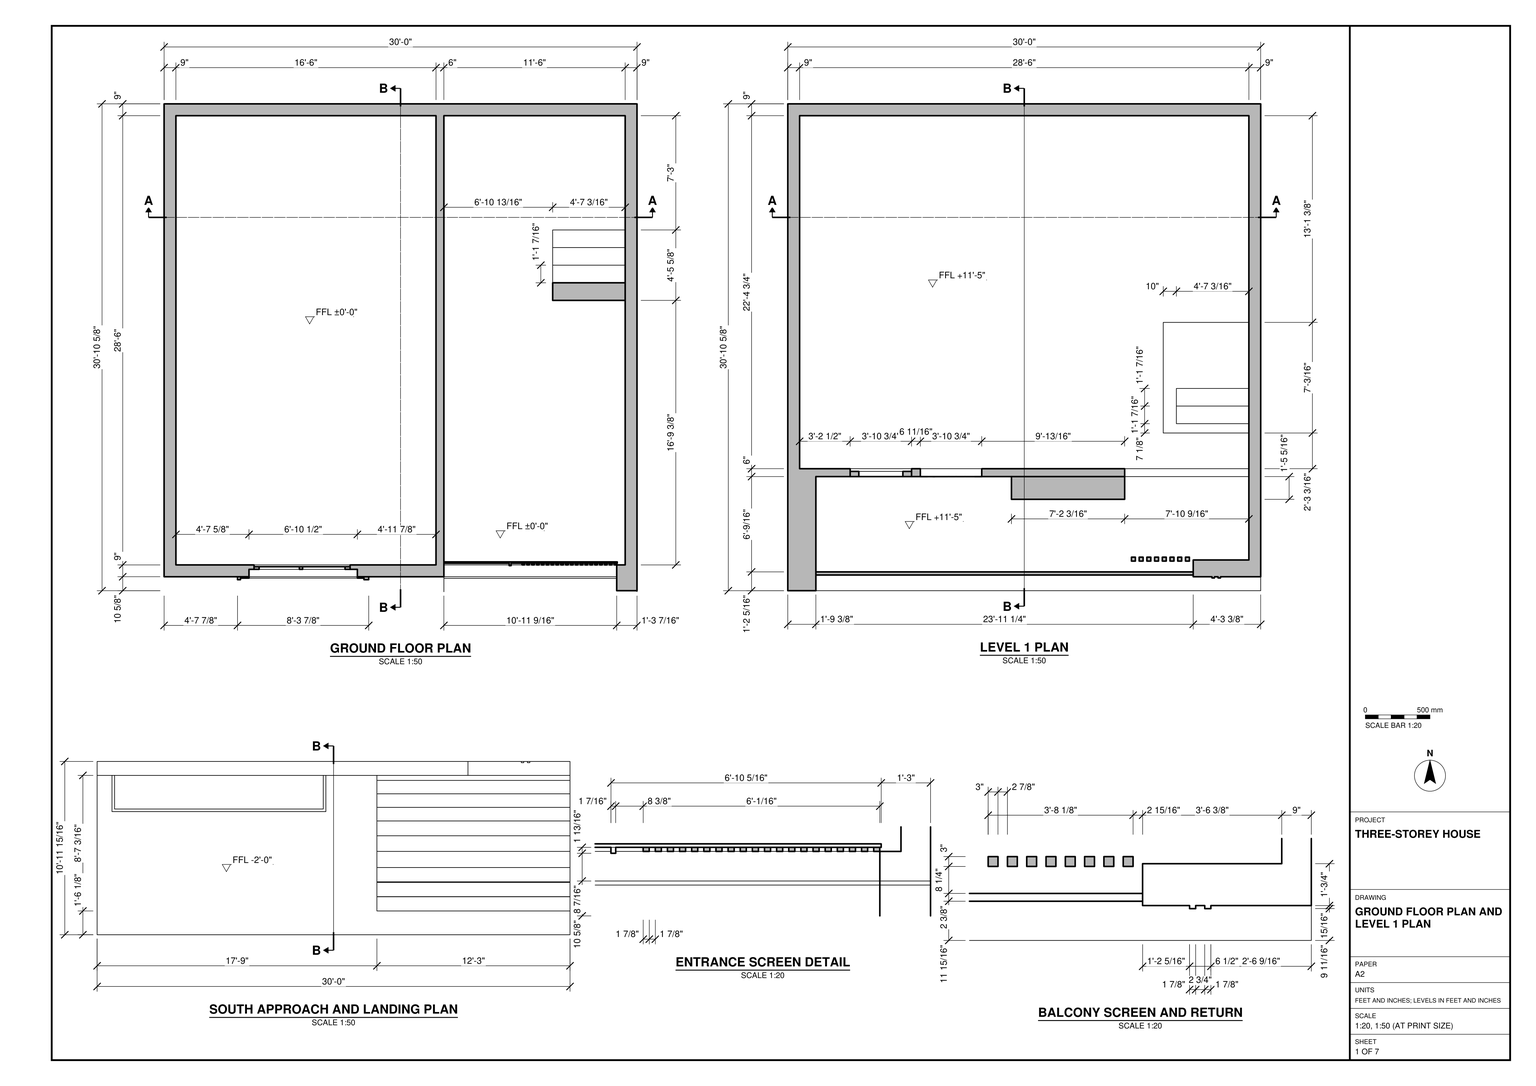
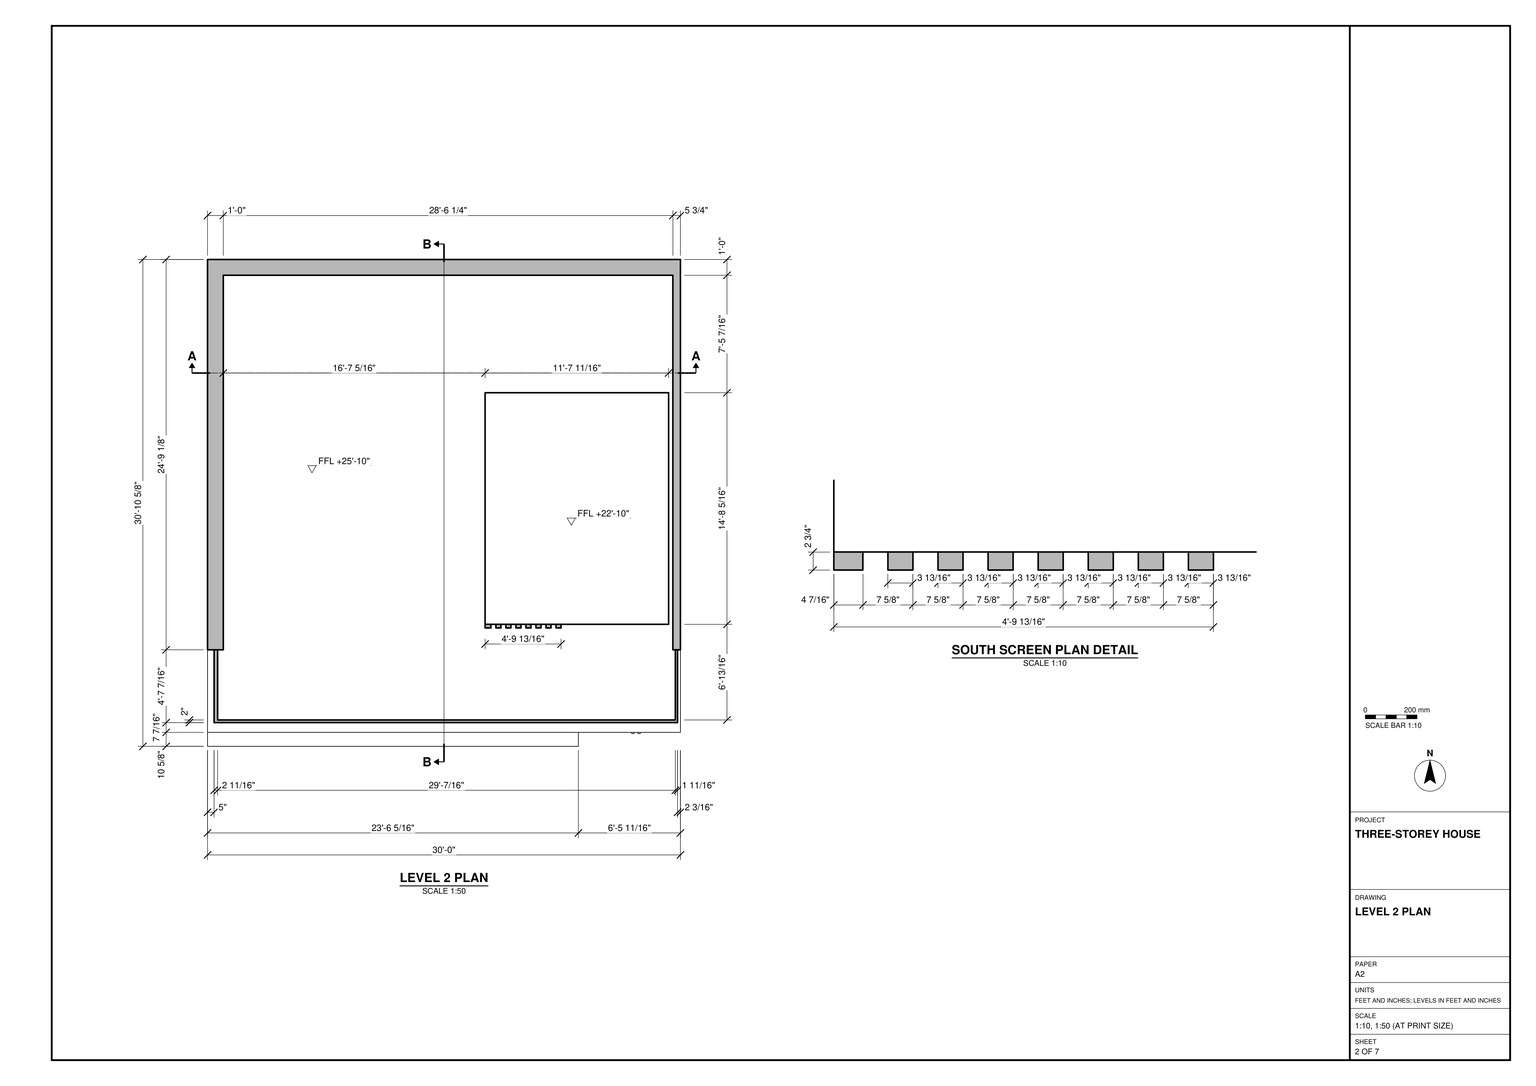
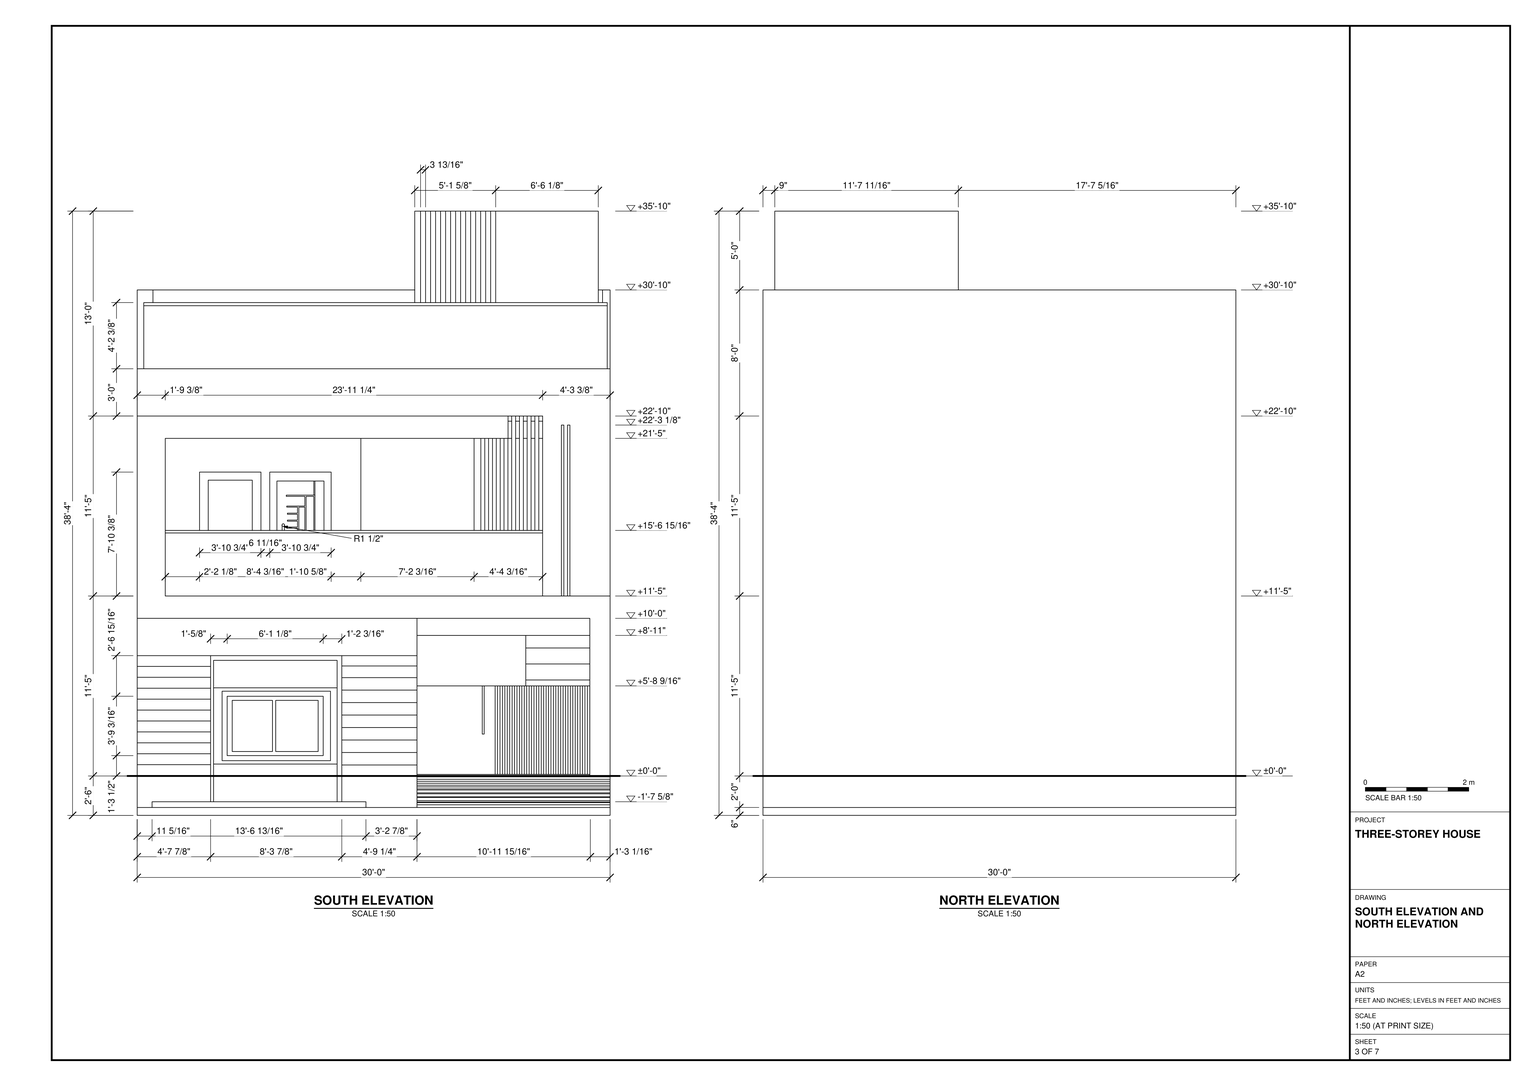
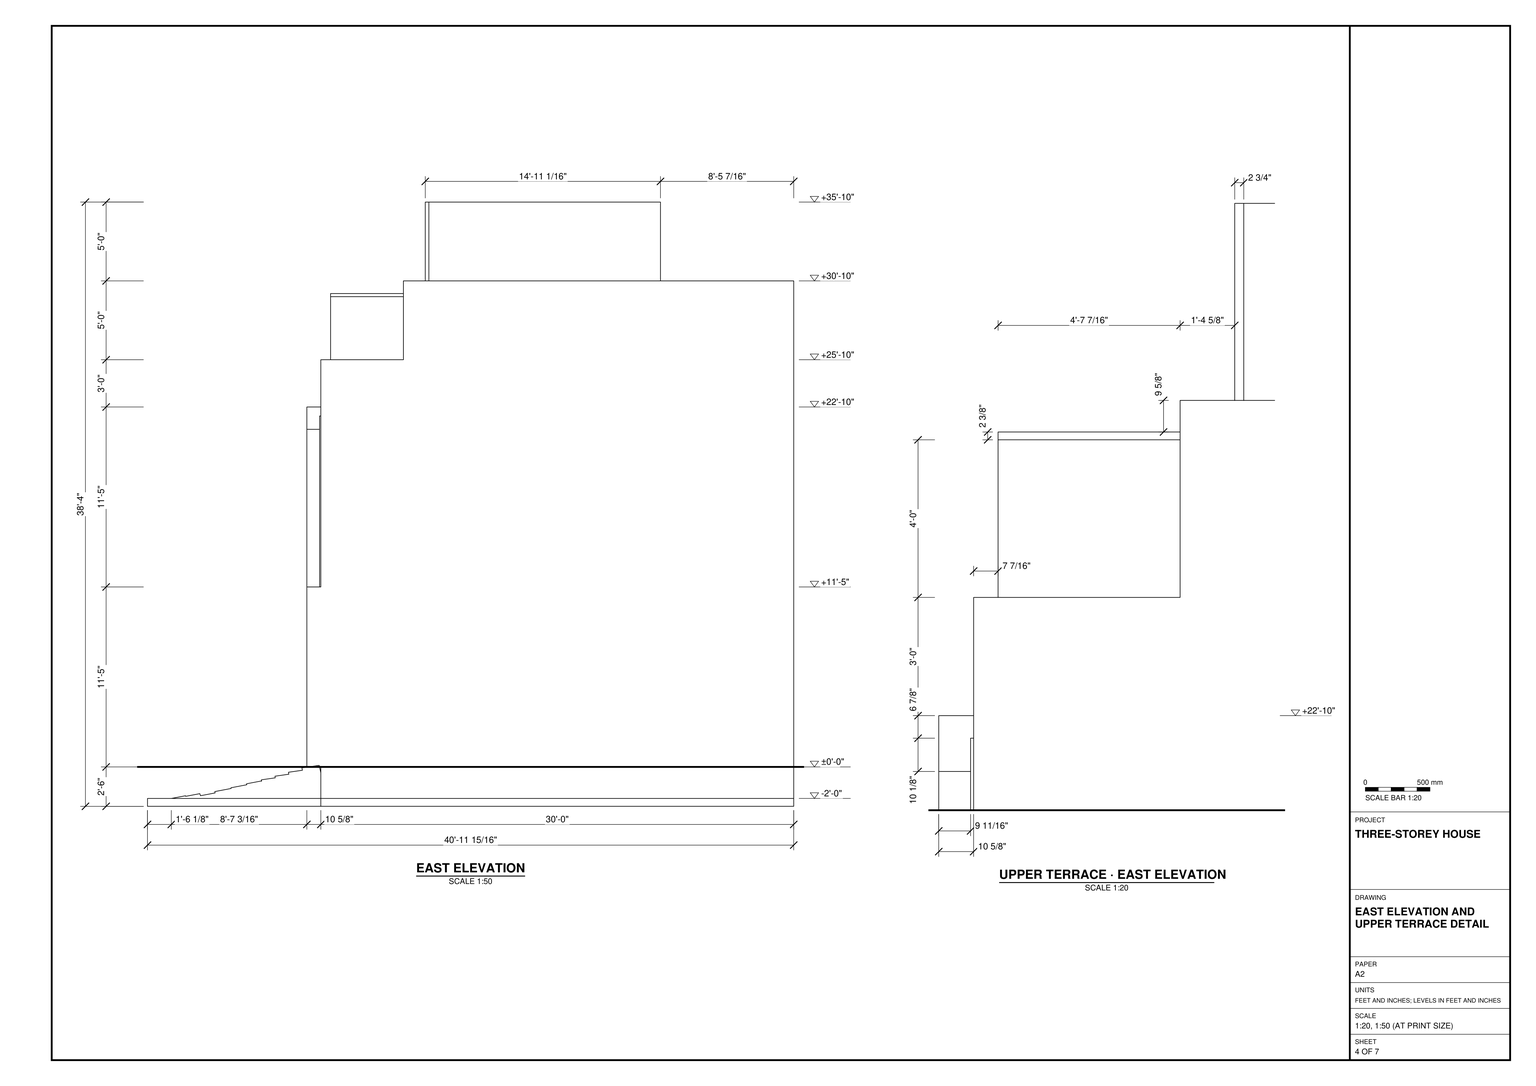
Build the three-storey house in SketchUp from task_files/diagram_01.pdf. Work in feet and inches. Including the south approach, make the model 30'-0" wide, 40'-11 15/16" deep and 38'-4" high. Set the finished floor levels at ±0'-0", +11'-5" and +22'-10".

Follow the plans for wall thicknesses, including the 9" ground-floor exterior walls and the 6" partition separating the wider west bay from the narrower east stair bay. Model the floor slabs, stair flights and landings. At the south approach, place the broad steps on the east side. Above them, form the entrance opening and its slatted screen; in the west bay, set the framed window into the horizontally banded wall.

Recess the Level 1 balcony behind the outer facade frame. Model the openings in its back wall and the screen and wall return at its east end. At Level 2, distinguish the raised terrace from the lower floor of the east enclosure. Follow the elevations for the flat roof, parapets and upper screen.

Keep walls, slabs, roof elements and any furniture or joinery pieces in separate groups or components, and use components for repeated parts. Decor and loose items shown may use any suitable library component. Save one SketchUp model as output_files/three_storey_house_with_a_recessed_south_balcony.skp.

# SketchUp Ruby script. Lengths in inches.
U = 1.inch
M = Sketchup.active_model
def pt(a) = Geom::Point3d.new(a.map { |v| v * U })
def face(e, loops, mat)
  f = e.add_face(loops[0].map { |a| pt(a) })
  loops[1..].each { |l| e.add_face(l.map { |a| pt(a) }).erase! }
  f.material = f.back_material = mat if mat
  f
end
# faces: each face lists its corners as indices into pts; further lists are holes
def faces(e, pts, list, mat = nil) = list.each { |f| face(e, (f[0].is_a?(Array) ? f : [f]).map { |l| l.map { |i| pts[i] } }, mat) }
# xy, xz, yz: faces in a plane at the given z, y or x. An outline is a flat list of corners, or four numbers for a rectangle; further outlines are holes
def ring(l) = l.size == 4 ? [[l[0], l[1]], [l[2], l[1]], [l[2], l[3]], [l[0], l[3]]] : l.each_slice(2).to_a
def flat(e, list, mat, &to3) = list.each { |f| face(e, (f[0].is_a?(Array) ? f : [f]).map { |l| ring(l).map { |u, v| to3.(u, v) } }, mat) }
def xy(e, z, list, mat = nil) = flat(e, list, mat) { |x, y| [x, y, z] }
def xz(e, y, list, mat = nil) = flat(e, list, mat) { |x, z| [x, y, z] }
def yz(e, x, list, mat = nil) = flat(e, list, mat) { |y, z| [x, y, z] }
def lines(e, pts, list) = list.each { |a, b| e.add_line(pt(pts[a]), pt(pts[b])) }
# prism: a flat outline (further loops are holes) pulled along v
def prism(e, loops, v, mat = nil)
  f = face(e, loops, mat); d = Geom::Vector3d.new(v.map { |x| x * U })
  f.pushpull(f.normal.samedirection?(d) ? d.length : -d.length)
end
def box(e, o, s, mat = nil) = prism(e, [[o, [o[0] + s[0], o[1], o[2]], [o[0] + s[0], o[1] + s[1], o[2]], [o[0], o[1] + s[1], o[2]]]], [0, 0, s[2]], mat)
def at(x, y, z, deg = 0) = Geom::Transformation.translation(pt([x, y, z])) * Geom::Transformation.rotation(ORIGIN, Z_AXIS, deg.degrees)
def axes(o, x, y, z) = Geom::Transformation.new([*x, 0, *y, 0, *z, 0, *pt(o).to_a, 1])
def part(name) = M.definitions.add(name)
# library, detail: a bought-in or finely detailed component or shape, given as its bounding box
def library(name, o, s) = part(name).tap { |d| box(d.entities, o, s) }
def detail(e, o, s) = box(e.add_group.entities, o, s)
def put(e, d, t, mat = nil) = e.add_instance(d, t).tap { |i| i.material = mat if mat }
def group(e, t, mat = nil) = e.add_group.tap { |g| g.transformation = t; g.material = mat if mat }.entities
root = M.entities
M.materials.add("[0116_Lavender]").color = [230, 230, 250]
M.materials.add("[0129_WhiteSmoke]").color = [245, 245, 245]
M.materials.add("[Color B08]").color = [57, 25, 0]
M.materials.add("[Color E01]").color = [255, 255, 204]
M.materials.add("[Color M00]").color = [255, 255, 255]
M.materials.add("[Color M02]").color = [198, 198, 198]
M.materials.add("[Color M06]").color = [86, 86, 86]
M.materials.add("[Color M07]").color = [58, 58, 58]
M.materials.add("[Grass Dark Green]").color = [106, 157, 55]
M.materials.add("[Groundcover Sand Smooth]").color = [182, 148, 101]
M.materials.add("[Metal Corrugated Shiny]").color = [193, 193, 171]
M.materials.add("[Translucent Glass Blue]").color = [108, 191, 246]
M.materials["[Translucent Glass Blue]"].alpha = 0.5
M.materials.add("[Translucent Glass Gray]").color = [128, 128, 128]
M.materials["[Translucent Glass Gray]"].alpha = 0.5
M.materials.add("[Wood Floor Parquet]").color = [145, 89, 39]
M.materials.add("[Wood Lumber ButtJoined]").color = [164, 152, 112]
M.materials.add("[Wood OSB]").color = [227, 195, 143]
M.materials.add("[Wood Plywood Knots]").color = [137, 122, 41]
M.materials.add("[Wood Veneer 01]").color = [67, 30, 37]
c1 = part("Group\#1")
box(c1.entities,[0,0,0],[55.1875,12,8])
xy(root,0,[[0,0,360,131.9375],[0,131.9375,360,491.9375]])
xy(root,6,[[55.875,129.6875,58.14,131.9375],[152.1875,129.6875,155.77,131.9375],[55.875,131.9375,55.875,134.0625,0,134.0625,0,491.9375,360,491.9375,360,131.9375,213,131.9375,213,134.875,155.77,134.875,155.77,131.9375]])
xy(root,6,[[[0,0,360,0,360,18.12,213,18.12,213,131.9375,155.77,131.9375,155.77,129.6875,152.1875,129.6875,152.1875,131.9375,58.14,131.9375,58.14,129.6875,55.875,129.6875,55.875,131.9375,0,131.9375],[11.33,93.75,174.14,125.88]],[0,131.9375,55.875,134.0625],[155.77,131.9375,213,134.875]],"[Color M00]")
xy(root,6,[[213,18.12,360,131.9375]],"[Color M02]")
xy(root,6,[[13.3,95.72,172.17,123.91]],"[Grass Dark Green]")
xy(root,10.375,[[[11.33,93.75,174.14,125.88],[13.3,95.72,172.17,123.91]]],"[Color M06]")
xy(root,30,[[344.5625,121.3125,360,131.9375],[0,131.9375,55.875,134.0625],[155.77,131.9375,213,134.875],[213,131.9375,344.5625,140.9375],[9,140.9375,207,482.9375],
  [213,140.9375,351,482.9375]])
xy(root,39.0625,[[58.14,130.875,152.1875,131.9375]])
xy(root,41.65,[[64.64,130.875,147.13,131.9375],[64.64,131.9375,147.13,137.5625]])
xy(root,45.49,[[68.48,137.5625,141.6,140.9375]])
xy(root,90.68,[[68.48,137.5625,141.6,140.9375]])
xy(root,94.52,[[64.64,130.875,147.13,131.9375],[64.64,131.9375,147.13,137.5625]])
xy(root,97.11,[[58.14,130.875,152.1875,131.9375]])
xy(root,118.02,[[58.14,129.6875,152.1875,131.9375]])
xy(root,121.6,[[55.875,129.6875,155.77,131.9375]])
xy(root,137,[[213,131.9375,344.5625,138.5625],[344.5625,138.5625,351,140.9375]])
xy(root,150,[[213,131.9375,351,138.5625],[213,138.5625,213,482.9375,285.8125,482.9375,285.8125,241.37,351,241.37,351,138.5625],[285.8125,325.5625,351,482.9375]])
xy(root,150,[[0,121.3125,213,131.9375],[213,121.3125,344.5625,131.9375]],"[Color M07]")
xy(root,162,[[9,140.9375,207,482.9375]])
xy(root,167,[[21.375,133.25,308.625,135.625],[[21.375,135.625,308.625,135.625,308.625,144.6875,351,144.6875,351,208.1875,256.44,208.1875,256.44,190.875,170.26,190.875,170.26,208.1875,147.65,208.1875,147.65,214.1875,100.91,214.1875,100.91,208.1875,94.21,208.1875,94.21,214.1875,47.47,214.1875,47.47,208.1875,21.375,208.1875],[261.6,143.85,264.6,146.85],[267.47,143.85,270.47,146.85],[273.35,143.85,276.35,146.85],[279.22,143.85,282.22,146.85],[285.1,143.85,288.1,146.85],[290.97,143.85,293.97,146.85],[296.85,143.85,299.85,146.85],[302.72,143.85,305.72,146.85]],[170.26,190.875,256.44,208.1875],[256.44,208.1875,351,214.1875],[9,214.1875,351,214.1875,351,241.37,285.8125,241.37,285.8125,325.5625,351,325.5625,351,482.9375,9,482.9375]])
xy(root,167,[[21.375,121.3125,360,121.3125,360,131.9375,329.41,131.9375,329.41,131,327.55,131,327.55,131.9375,324.79,131.9375,324.79,131,322.93,131,322.93,131.9375,308.625,131.9375,308.625,133.25,21.375,133.25],[261.6,143.85,264.6,146.85],[267.47,143.85,270.47,146.85],[273.35,143.85,276.35,146.85],[279.22,143.85,282.22,146.85],
  [285.1,143.85,288.1,146.85],[290.97,143.85,293.97,146.85],[296.85,143.85,299.85,146.85],[302.72,143.85,305.72,146.85]],"[Color M07]")
xy(root,215,[[21.375,133.25,308.625,135.625]])
xy(root,216.9375,[[21.375,133.25,308.625,135.625]],"[Color M07]")
xy(root,261.34,[[47.47,208.1875,94.21,214.1875],[100.91,208.1875,147.65,214.1875]])
xy(root,287,[[9,140.9375,21.375,208.1875],[170.26,190.875,256.44,208.1875],[256.44,190.875,282.32,208.1875],[256.44,208.1875,282.32,214.1875]])
xy(root,287,[[[21.375,121.3125,21.375,208.1875,170.26,208.1875,170.26,190.875,282.32,190.875,282.32,121.3125],[279.22,143.85,282.22,146.85],[273.35,143.85,276.35,146.85],[267.47,143.85,270.47,146.85],[261.6,143.85,264.6,146.85]]],"[Wood Plywood Knots]")
xy(root,297.14,[[322.93,131,324.79,131.9375],[327.55,131,329.41,131.9375]],"[0129_WhiteSmoke]")
xy(root,300.0625,[[9,214.1875,351,482.9375]])
xy(root,304,[[9,131.9375,282.32,208.1875],[282.32,131.9375,282.32,208.1875,351,208.1875,351,144.6875,308.625,144.6875,308.625,131.9375,305.72,131.9375,305.72,146.85,302.72,146.85,302.72,131.9375,299.85,131.9375,299.85,146.85,296.85,146.85,296.85,131.9375,293.97,131.9375,293.97,146.85,290.97,146.85,290.97,131.9375,288.1,131.9375,288.1,146.85,285.1,146.85,285.1,131.9375],[285.1,131.9375,288.1,143.85],[290.97,131.9375,293.97,143.85],[296.85,131.9375,299.85,143.85],
  [302.72,131.9375,305.72,143.85],[282.32,208.1875,351,214.1875],[9,214.1875,351,482.9375]])
xy(root,304,[[0,121.3125,282.32,131.9375],[285.1,143.85,288.1,146.85],[290.97,143.85,293.97,146.85],[296.85,143.85,299.85,146.85],[302.72,143.85,305.72,146.85]],"[Color M07]")
xy(root,334,[[9,214.1875,351,482.9375]])
xy(root,340,[[0,131.9375,360,131.9375,360,194.81,357.8125,194.81,357.8125,139.375,5,139.375,5,194.81,0,194.81],[5,139.375,5,194.81,7.6875,194.81,7.6875,141.375,356.125,141.375,356.125,194.81,357.8125,194.81,357.8125,139.375],[[7.6875,141.375,356.125,141.375,356.125,194.81,354.25,194.81,354.25,479.9375,12,479.9375,12,194.81,7.6875,194.81],[211.29,211.4375,211.29,390.5,351,390.5,351,214.1875,269.09,214.1875,269.09,211.4375,265.27,211.4375,265.27,214.1875,261.46,214.1875,261.46,211.4375,257.65,211.4375,257.65,214.1875,253.84,214.1875,253.84,211.4375,250.02,211.4375,250.02,214.1875,246.21,214.1875,246.21,211.4375,242.4,211.4375,242.4,214.1875,238.59,214.1875,238.59,211.4375,234.77,211.4375,234.77,214.1875,230.96,214.1875,230.96,211.4375,227.15,211.4375,227.15,214.1875,223.34,214.1875,223.34,211.4375,219.52,211.4375,219.52,214.1875,215.71,214.1875,215.71,211.4375]],[211.29,214.1875,351,390.5]])
xy(root,340,[[211.29,211.4375,215.71,214.1875],[219.52,211.4375,223.34,214.1875],[227.15,211.4375,230.96,214.1875],[234.77,211.4375,238.59,214.1875],[242.4,211.4375,246.21,214.1875],
  [250.02,211.4375,253.84,214.1875],[257.65,211.4375,261.46,214.1875],[265.27,211.4375,269.09,214.1875]],"[Color M07]")
xy(root,388,[[5,139.375,5,194.81,7.6875,194.81,7.6875,141.375,356.125,141.375,356.125,194.81,357.8125,194.81,357.8125,139.375]])
xy(root,390.375,[[5,139.375,357.8125,139.375,357.8125,194.81,356.125,194.81,356.125,141.375,7.6875,141.375,7.6875,194.81,5,194.81]],"[Color M07]")
xy(root,400,[[0,194.81,12,194.81,12,479.9375,354.25,479.9375,354.25,194.81,360,194.81,360,491.9375,0,491.9375]])
xy(root,460,[[211.29,211.4375,215.71,214.1875],[219.52,211.4375,223.34,214.1875],[227.15,211.4375,230.96,214.1875],[234.77,211.4375,238.59,214.1875],[242.4,211.4375,246.21,214.1875],
  [250.02,211.4375,253.84,214.1875],[257.65,211.4375,261.46,214.1875],[265.27,211.4375,269.09,214.1875]],"[Color M07]")
xy(root,460,[[211.29,214.1875,351,390.5]],"[Wood Lumber ButtJoined]")
xz(root,0,[[0,0,360,6]])
xz(root,93.75,[[11.33,6,174.14,10.375]],"[Color M06]")
xz(root,95.72,[[13.3,6,172.17,10.375]],"[Color M06]")
xz(root,121.3125,[[344.5625,30,360,30,360,167,21.375,167,21.375,287,282.32,287,282.32,304,0,304,0,150,344.5625,150]],"[Color M07]")
xz(root,123.91,[[13.3,6,172.17,10.375]],"[Color M06]")
xz(root,125.88,[[11.33,6,174.14,10.375]],"[Color M06]")
xz(root,129.6875,[[55.875,6,58.14,6,58.14,118.02,152.1875,118.02,152.1875,6,155.77,6,155.77,121.6,55.875,121.6]])
xz(root,130.875,[[[58.14,39.0625,152.1875,97.11],[64.64,41.65,147.13,94.52]]])
xz(root,131,[[322.93,167,324.79,297.14],[327.55,167,329.41,297.14]],"[0129_WhiteSmoke]")
xz(root,131.9375,[[0,0,360,6],[55.875,6,55.875,121.6,155.77,121.6,155.77,6,152.1875,6,152.1875,118.02,58.14,118.02,58.14,97.11,59.46,97.11,59.46,39.0625,58.14,39.0625,58.14,6],[213,25.44,360,30],[0,30,55.875,38.6],[155.77,30,213,38.36],
  [155.77,38.36,213,47.86],[0,38.6,55.875,46.91],[[59.46,39.0625,152.1875,97.11],[64.64,41.65,147.13,94.52]],[0,46.91,55.875,55.22],[155.77,47.86,213,57.36],
  [0,55.22,55.875,63.54],[155.77,57.36,213,66.86],[0,63.54,55.875,71.85],[155.77,66.86,213,76.36],[0,71.85,55.875,80.16],
  [155.77,76.36,213,85.86],[0,80.16,55.875,88.47],[155.77,85.86,213,95.36],[0,88.47,55.875,96.79],[155.77,95.36,213,104.86],
  [0,96.79,55.875,105.1],[155.77,104.86,213,113.74],[0,105.1,55.875,113.41],[0,113.41,55.875,121.6],[155.77,113.74,213,121.6],
  [213,137,344.5625,150]])
xz(root,131.9375,[[308.625,167,322.93,167,322.93,297.14,324.79,297.14,324.79,167,327.55,167,327.55,297.14,329.41,297.14,329.41,167,360,167,360,340,0,340,0,304,308.625,304]],"[0116_Lavender]")
xz(root,131.9375,[[213,6,360,25.44]],"[Color M02]")
xz(root,131.9375,[[0,121.6,213,150]],"[Wood Floor Parquet]")
xz(root,131.9375,[[58.14,6,152.1875,39.0625],[58.14,97.11,152.1875,118.02]],"[Wood OSB]")
xz(root,133.25,[[21.375,215,308.625,216.9375]],"[Color M07]")
xz(root,133.25,[[21.375,167,308.625,215]],"[Translucent Glass Gray]")
xz(root,134.0625,[[0,6,55.875,30]],"[Groundcover Sand Smooth]")
xz(root,134.875,[[155.77,6,213,30]],"[Groundcover Sand Smooth]")
xz(root,135.625,[[21.375,215,308.625,216.9375]],"[Color M07]")
xz(root,135.625,[[21.375,167,308.625,215]],"[Translucent Glass Gray]")
xz(root,137.5625,[[[64.64,41.65,147.13,94.52],[68.48,45.49,141.6,90.68]]])
xz(root,138.5625,[[213,137,351,150]])
xz(root,139.375,[[5,388,357.8125,390.375]],"[Color M07]")
xz(root,139.375,[[5,340,357.8125,388]],"[Translucent Glass Blue]")
xz(root,140.9375,[[[9,30,207,150],[68.48,45.49,141.6,90.68]],[344.5625,30,351,137],[9,150,207,162],[9,162,20.5625,167]])
xz(root,141.375,[[7.6875,388,356.125,390.375]],"[Color M07]")
xz(root,141.375,[[7.6875,340,356.125,388]],"[Translucent Glass Blue]")
xz(root,143.85,[[261.6,167,264.6,287],[267.47,167,270.47,287],[273.35,167,276.35,287],[279.22,167,282.22,287],[285.1,167,288.1,304],
  [290.97,167,293.97,304],[296.85,167,299.85,304],[302.72,167,305.72,304]],"[Color M07]")
xz(root,144.6875,[[308.625,167,351,304]])
xz(root,146.85,[[261.6,167,264.6,287],[267.47,167,270.47,287],[273.35,167,276.35,287],[279.22,167,282.22,287],[285.1,167,288.1,304],
  [290.97,167,293.97,304],[296.85,167,299.85,304],[302.72,167,305.72,304]],"[Color M07]")
xz(root,190.875,[[170.26,167,256.44,287]],"[Wood Floor Parquet]")
xz(root,194.81,[[0,340,5,340,5,390.375,7.6875,390.375,7.6875,340,12,340,12,400,0,400],[5,340,7.6875,388],[354.25,340,356.125,340,356.125,390.375,357.8125,390.375,357.8125,340,360,340,360,400,354.25,400],[356.125,340,357.8125,388],[5,388,7.6875,390.375],
  [356.125,388,357.8125,390.375]])
xz(root,208.1875,[[170.26,167,256.44,287],[9,287,282.32,304]])
xz(root,208.1875,[[21.375,167,47.47,167,47.47,261.34,94.21,261.34,94.21,167,100.91,167,100.91,261.34,147.65,261.34,147.65,167,170.26,167,170.26,287,21.375,287]],"[Color E01]")
xz(root,211.4375,[[211.29,340,215.71,460],[219.52,340,223.34,460],[227.15,340,230.96,460],[234.77,340,238.59,460],[242.4,340,246.21,460],
  [250.02,340,253.84,460],[257.65,340,261.46,460],[265.27,340,269.09,460]],"[Color M07]")
xz(root,214.1875,[[9,167,9,287,256.44,287,256.44,167,147.65,167,147.65,261.34,100.91,261.34,100.91,167,94.21,167,94.21,261.34,47.47,261.34,47.47,167],[9,287,282.32,300.0625],[9,300.0625,282.32,304],[282.32,300.0625,351,304],[9,304,351,334],
  [333,334,351,340]])
xz(root,214.1875,[[211.29,340,215.71,460],[215.71,340,219.52,460],[219.52,340,223.34,460],[223.34,340,227.15,460],[227.15,340,230.96,460],
  [230.96,340,234.77,460],[234.77,340,238.59,460],[238.59,340,242.4,460],[242.4,340,246.21,460],[246.21,340,250.02,460],
  [250.02,340,253.84,460],[253.84,340,257.65,460],[257.65,340,261.46,460],[261.46,340,265.27,460],[265.27,340,269.09,460],
  [269.09,340,272.9,460]],"[Color M07]")
xz(root,214.1875,[[272.9,340,351,460]],"[Wood Lumber ButtJoined]")
xz(root,241.37,[[285.8125,150,351,167]])
xz(root,325.5625,[[285.8125,150,351,167]])
xz(root,390.5,[[211.29,340,351,460]],"[Wood Lumber ButtJoined]")
xz(root,479.9375,[[12,340,354.25,400]])
xz(root,482.9375,[[9,30,207,150],[213,30,351,150],[9,150,207,162],[9,162,207,167],[9,167,207,287],
  [207,167,351,287],[9,287,207,300.0625],[207,287,351,300.0625],[9,300.0625,207,304],[207,300.0625,351,304],
  [9,304,207,334],[207,304,351,334]])
xz(root,491.9375,[[0,0,360,6],[0,6,360,400]])
yz(root,0,[[0,0,131.9375,6],[131.9375,0,491.9375,6],[134.0625,6,134.0625,30,131.9375,30,131.9375,150,121.3125,150,121.3125,304,131.9375,304,131.9375,340,194.81,340,194.81,400,491.9375,400,491.9375,6]])
yz(root,5,[[139.375,388,194.81,390.375]],"[Color M07]")
yz(root,5,[[139.375,340,194.81,388]],"[Translucent Glass Blue]")
yz(root,7.6875,[[141.375,340,194.81,388]])
yz(root,7.6875,[[141.375,388,194.81,390.375]],"[Color M07]")
yz(root,9,[[140.9375,30,482.9375,150],[140.9375,150,482.9375,162],[214.1875,167,482.9375,287],[214.1875,287,482.9375,300.0625],[214.1875,300.0625,232.1875,304],
  [232.1875,300.0625,482.9375,304],[214.1875,304,482.9375,334]])
yz(root,11.33,[[93.75,6,125.88,10.375]],"[Color M06]")
yz(root,12,[[194.81,340,479.9375,400]])
yz(root,13.3,[[95.72,6,123.91,10.375]],"[Color M06]")
yz(root,21.375,[[133.25,167,135.625,215],[133.25,215,135.625,216.9375]])
yz(root,21.375,[[121.3125,167,133.25,167,133.25,216.9375,135.625,216.9375,135.625,167,208.1875,167,208.1875,287,121.3125,287]],"[Color M07]")
yz(root,47.47,[[208.1875,167,214.1875,261.34]])
yz(root,55.875,[[129.6875,6,131.9375,30],[131.9375,6,134.0625,30],[129.6875,30,131.9375,121.6]])
yz(root,58.14,[[129.6875,6,131.9375,6,131.9375,39.0625,130.875,39.0625,130.875,97.11,131.9375,97.11,131.9375,118.02,129.6875,118.02]])
yz(root,64.64,[[130.875,41.65,131.9375,94.52],[131.9375,41.65,137.5625,94.52]])
yz(root,68.48,[[137.5625,45.49,140.9375,90.68]])
yz(root,94.21,[[208.1875,167,214.1875,261.34]])
yz(root,100.91,[[208.1875,167,214.1875,261.34]])
yz(root,141.6,[[137.5625,45.49,140.9375,90.68]])
yz(root,147.13,[[130.875,41.65,131.9375,94.52],[131.9375,41.65,137.5625,94.52]])
yz(root,147.65,[[208.1875,167,214.1875,261.34]])
yz(root,152.1875,[[129.6875,6,129.6875,118.02,131.9375,118.02,131.9375,97.11,130.875,97.11,130.875,39.0625,131.9375,39.0625,131.9375,6]])
yz(root,155.77,[[129.6875,6,131.9375,30],[131.9375,6,134.875,30],[129.6875,30,131.9375,121.6]])
yz(root,170.26,[[190.875,167,208.1875,287]],"[Wood Floor Parquet]")
yz(root,172.17,[[95.72,6,123.91,10.375]],"[Color M06]")
yz(root,174.14,[[93.75,6,125.88,10.375]],"[Color M06]")
yz(root,207,[[140.9375,30,482.9375,150],[140.9375,150,482.9375,162]])
yz(root,211.29,[[211.4375,340,214.1875,460]],"[Color M07]")
yz(root,211.29,[[214.1875,340,390.5,460]],"[Wood Lumber ButtJoined]")
yz(root,213,[[131.9375,6,134.875,30],[131.9375,30,482.9375,30,482.9375,150,138.5625,150,138.5625,137,131.9375,137],[131.9375,137,138.5625,150]])
yz(root,213,[[18.12,6,28.91,8.05,29.04,7.6,39.84,9.65,40.3,8.07,51.49,10.19,51.1875,11.22,63.63,13.58,63.47,14.125,75.57,16.42,75.36,17.16,86.79,19.32,86.87,19.02,86.625,20.17,97.26,21.69,96.98,22.93,107.62,24.45,107.29,25.94,117.91,27.45,117.51,29.3,130.69,31.17,131.9375,25.44,131.9375,6]],"[Color M02]")
yz(root,215.71,[[211.4375,340,214.1875,460]],"[Color M07]")
yz(root,219.52,[[211.4375,340,214.1875,460]],"[Color M07]")
yz(root,223.34,[[211.4375,340,214.1875,460]],"[Color M07]")
yz(root,227.15,[[211.4375,340,214.1875,460]],"[Color M07]")
yz(root,230.96,[[211.4375,340,214.1875,460]],"[Color M07]")
yz(root,234.77,[[211.4375,340,214.1875,460]],"[Color M07]")
yz(root,238.59,[[211.4375,340,214.1875,460]],"[Color M07]")
yz(root,242.4,[[211.4375,340,214.1875,460]],"[Color M07]")
yz(root,246.21,[[211.4375,340,214.1875,460]],"[Color M07]")
yz(root,250.02,[[211.4375,340,214.1875,460]],"[Color M07]")
yz(root,253.84,[[211.4375,340,214.1875,460]],"[Color M07]")
yz(root,256.44,[[190.875,167,208.1875,287],[208.1875,167,214.1875,287]])
yz(root,257.65,[[211.4375,340,214.1875,460]],"[Color M07]")
yz(root,261.46,[[211.4375,340,214.1875,460]],"[Color M07]")
yz(root,261.6,[[143.85,167,146.85,287]],"[Color M07]")
yz(root,264.6,[[143.85,167,146.85,287]],"[Color M07]")
yz(root,265.27,[[211.4375,340,214.1875,460]],"[Color M07]")
yz(root,267.47,[[143.85,167,146.85,287]],"[Color M07]")
yz(root,269.09,[[211.4375,340,214.1875,460]],"[Color M07]")
yz(root,270.47,[[143.85,167,146.85,287]],"[Color M07]")
yz(root,273.35,[[143.85,167,146.85,287]],"[Color M07]")
yz(root,276.35,[[143.85,167,146.85,287]],"[Color M07]")
yz(root,279.22,[[143.85,167,146.85,287]],"[Color M07]")
yz(root,282.22,[[143.85,167,146.85,287]],"[Color M07]")
yz(root,282.32,[[121.3125,287,208.1875,304],[208.1875,287,214.1875,304]])
yz(root,285.1,[[143.85,167,146.85,304]],"[Color M07]")
yz(root,285.8125,[[241.37,150,325.5625,167]])
yz(root,288.1,[[143.85,167,146.85,304]],"[Color M07]")
yz(root,290.97,[[143.85,167,146.85,304]],"[Color M07]")
yz(root,293.97,[[143.85,167,146.85,304]],"[Color M07]")
yz(root,296.85,[[143.85,167,146.85,304]],"[Color M07]")
yz(root,299.85,[[143.85,167,146.85,304]],"[Color M07]")
yz(root,302.72,[[143.85,167,146.85,304]],"[Color M07]")
yz(root,305.72,[[143.85,167,146.85,304]],"[Color M07]")
yz(root,308.625,[[131.9375,167,131.9375,304,144.6875,304,144.6875,167,135.625,167,135.625,216.9375,133.25,216.9375,133.25,167],[133.25,167,135.625,215],[133.25,215,135.625,216.9375]])
yz(root,322.93,[[131,167,131.9375,297.14]],"[0129_WhiteSmoke]")
yz(root,324.79,[[131,167,131.9375,297.14]],"[0129_WhiteSmoke]")
yz(root,327.55,[[131,167,131.9375,297.14]],"[0129_WhiteSmoke]")
yz(root,329.41,[[131,167,131.9375,297.14]],"[0129_WhiteSmoke]")
yz(root,344.5625,[[121.3125,30,121.3125,150,131.9375,150,131.9375,137,140.9375,137,140.9375,30]],"[Color M07]")
yz(root,351,[[241.37,150,325.5625,167],[144.6875,167,208.1875,304],[208.1875,167,214.1875,287],[214.1875,167,241.37,287],[241.37,167,325.5625,287],
  [325.5625,167,482.9375,287],[208.1875,287,214.1875,304],[214.1875,287,241.37,300.0625],[241.37,287,325.5625,300.0625],[325.5625,287,482.9375,300.0625],
  [214.1875,300.0625,241.37,304],[241.37,300.0625,325.5625,304],[325.5625,300.0625,482.9375,304],[214.1875,304,241.37,334],[241.37,304,325.5625,334],
  [325.5625,304,482.9375,334],[214.1875,334,241.37,340],[241.37,334,325.5625,340]])
yz(root,351,[[214.1875,340,390.5,460]],"[Wood Lumber ButtJoined]")
yz(root,351,[[140.9375,30,140.9375,137,138.5625,137,138.5625,150,482.9375,150,482.9375,30]],"[Wood OSB]")
yz(root,354.25,[[194.81,340,478.56,400],[478.56,340,479.9375,400]])
yz(root,356.125,[[141.375,388,194.81,390.375]],"[Color M07]")
yz(root,356.125,[[141.375,340,194.81,388]],"[Translucent Glass Blue]")
yz(root,357.8125,[[139.375,388,194.81,390.375]],"[Color M07]")
yz(root,357.8125,[[139.375,340,194.81,388]],"[Translucent Glass Blue]")
yz(root,360,[[0,0,131.9375,6],[131.9375,0,491.9375,6],[131.9375,6,491.9375,6,491.9375,400,194.81,400,194.81,340,131.9375,340,131.9375,167,121.3125,167,121.3125,30,122.45,30,130.69,31.17,130.95,30,131.9375,30],[122.45,30,130.95,30,130.69,31.17]])
yz(root,360,[[18.12,6,131.9375,6,131.9375,25.44,130.95,30,122.45,30,117.51,29.3,117.91,27.45,107.29,25.94,107.62,24.45,96.98,22.93,97.26,21.69,86.625,20.17,86.87,19.02,86.79,19.32,75.36,17.16,75.57,16.42,63.47,14.125,63.63,13.58,51.1875,11.22,51.49,10.19,40.3,8.07,39.84,9.65,29.04,7.6,28.91,8.05]],"[Color M02]")
# 8 loose lines left out
p = [[360,18.12,6],[360,28.91,8.05],[213,28.91,8.05],[213,18.12,6],[213,29.04,7.6],[360,29.04,7.6],
  [213,39.84,9.65],[360,39.84,9.65],[213,40.3,8.07],[360,40.3,8.07],[213,51.49,10.19],[360,51.49,10.19],
  [213,51.1875,11.22],[360,51.1875,11.22],[213,63.63,13.58],[360,63.63,13.58],[213,63.47,14.125],[360,63.47,14.125],
  [213,75.57,16.42],[360,75.57,16.42],[213,75.36,17.16],[360,75.36,17.16],[213,86.79,19.32],[360,86.79,19.32],
  [213,86.87,19.02],[360,86.87,19.02],[360,86.625,20.17],[213,86.625,20.17],[360,97.26,21.69],[213,97.26,21.69],
  [213,96.98,22.93],[360,96.98,22.93],[213,107.62,24.45],[360,107.62,24.45],[213,107.29,25.94],[360,107.29,25.94],
  [360,131.9375,25.44],[213,131.9375,25.44],[213,130.69,31.17],[360,130.69,31.17],[360,130.95,30],[213,117.91,27.45],
  [360,117.91,27.45],[213,117.51,29.3],[360,117.51,29.3],[360,122.45,30]]
faces(root,p,[[0,1,2,3],[6,4,5,7],[10,8,9,11],[12,10,11,13],[14,12,13,15],[16,14,15,17],[18,16,17,19],[20,18,19,21],
  [22,20,21,23],[24,25,26,27],[26,28,29,27],[30,29,28,31],[32,30,31,33],[34,32,33,35],[36,37,38,39,40],[41,34,35,42],
  [43,41,42,44],[38,43,44,45,39]],"[Color M02]")
faces(root,p,[[4,2,1,5],[8,6,7,9],[25,24,22,23]])
g1 = group(root,at(295.8125,248.47,30))
put(g1,c1,axes([0,40.22,85.26],[1,0,0],[0,1.1172,0],[0,0,1.5225]))
g2 = group(g1,at(55.1875,147.47,0))
put(g2,c1,axes([0,-80.4375,73.08],[-1,0,0],[0,-1.1172,0],[0,0,1.5225]))
put(g2,c1,axes([0,0,0],[-1,0,0],[0,-1.1172,0],[0,0,1.5225]))
put(g2,c1,axes([0,-13.41,12.18],[-1,0,0],[0,-1.1172,0],[0,0,1.5225]))
put(g2,c1,axes([0,-26.8125,24.36],[-1,0,0],[0,-1.1172,0],[0,0,1.5225]))
put(g2,c1,axes([0,-53.625,48.72],[-1,0,0],[0,-1.1172,0],[0,0,1.5225]))
put(g2,c1,axes([0,-40.22,36.54],[-1,0,0],[0,-1.1172,0],[0,0,1.5225]))
put(g2,c1,axes([0,-67.03,60.9],[-1,0,0],[0,-1.1172,0],[0,0,1.5225]))
put(g1,c1,axes([0,26.8125,97.44],[1,0,0],[0,1.1172,0],[0,0,1.5225]))
put(g1,c1,axes([0,13.41,109.62],[1,0,0],[0,1.1172,0],[0,0,1.5225]))
put(g1,c1,axes([0,0,121.8],[1,0,0],[0,1.1172,0],[0,0,1.5225]))
g3 = group(root,at(47.47,208.1875,167))
xy(g3,0,[[0,0,46.74,3.9375]],"[Color B08]")
xy(g3,6.16,[[6.61,0,40.13,3.9375]],"[Color B08]")
xy(g3,88.1875,[[6.61,0,40.13,3.9375]],"[Color B08]")
xy(g3,94.34,[[0,0,46.74,3.9375]],"[Color B08]")
xz(g3,0,[[[0,0,46.74,94.34],[6.61,6.16,40.13,88.1875]]],"[Color B08]")
xz(g3,0,[[6.61,6.16,40.13,88.1875]],"[Translucent Glass Gray]")
xz(g3,3.9375,[[[0,0,46.74,94.34],[6.61,6.16,40.13,88.1875]]],"[Color B08]")
yz(g3,0,[[0,0,3.9375,94.34]],"[Color B08]")
yz(g3,6.61,[[0,6.16,3.9375,88.1875]],"[Color B08]")
yz(g3,40.13,[[0,6.16,3.9375,88.1875]],"[Color B08]")
yz(g3,46.74,[[0,0,3.9375,94.34]],"[Color B08]")
g4 = group(root,at(100.91,208.125,167))
xy(g4,0,[[0,0,46.74,0.0625]],"[Wood Veneer 01]")
xy(g4,6.81,[[5.45,0,41.28,0.03],[5.45,0.03,41.28,0.0625]],"[Wood Veneer 01]")
xy(g4,11.67,[[26.72,0.03,27.66,0.0625]],"[Wood Veneer 01]")
xy(g4,11.88,[[33.5625,0.03,34.41,0.0625]],"[Wood Veneer 01]")
xy(g4,12.18,[[21.11,0.03,22.15,0.0625]],"[Wood Veneer 01]")
xy(g4,23.79,[[13.46,0.03,21.11,0.0625]],"[Wood Veneer 01]")
xy(g4,24.64,[[13.46,0.03,21.11,0.0625]],"[Wood Veneer 01]")
xy(g4,30.49,[[13.46,0.03,21.11,0.0625]],"[Wood Veneer 01]")
xy(g4,31.34,[[13.46,0.03,21.11,0.0625]],"[Wood Veneer 01]")
xy(g4,35.78,[[13.46,0.03,21.11,0.0625]],"[Wood Veneer 01]")
xy(g4,36.63,[[13.46,0.03,21.11,0.0625]],"[Wood Veneer 01]")
xy(g4,41.07,[[13.46,0.03,21.11,0.0625]],"[Wood Veneer 01]")
xy(g4,41.92,[[13.46,0.03,21.11,0.0625]],"[Wood Veneer 01]")
xy(g4,46.36,[[13.46,0.03,21.11,0.0625]],"[Wood Veneer 01]")
xy(g4,47.21,[[13.46,0.03,21.11,0.0625]],"[Wood Veneer 01]")
xy(g4,51.65,[[13.46,0.03,21.11,0.0625]],"[Wood Veneer 01]")
xy(g4,52.5,[[13.46,0.03,21.11,0.0625]],"[Wood Veneer 01]")
xy(g4,56.9375,[[13.46,0.03,21.11,0.0625]],"[Wood Veneer 01]")
xy(g4,57.79,[[13.46,0.03,21.11,0.0625]],"[Wood Veneer 01]")
xy(g4,62.23,[[13.46,0.03,21.11,0.0625]],"[Wood Veneer 01]")
xy(g4,63.08,[[13.46,0.03,21.11,0.0625]],"[Wood Veneer 01]")
xy(g4,67.67,[[12.97,0.03,21.11,0.0625],[22.15,0.03,26.72,0.0625]],"[Wood Veneer 01]")
xy(g4,68.49,[[12.97,0.03,26.72,0.0625]],"[Wood Veneer 01]")
xy(g4,75.86,[[12.58,0.03,26.72,0.0625],[27.66,0.03,33.5625,0.0625]],"[Wood Veneer 01]")
xy(g4,76.8,[[12.58,0.03,33.5625,0.0625],[33.5625,0.03,34.41,0.0625]],"[Wood Veneer 01]")
xy(g4,87.54,[[5.45,0,33.5625,0.03],[33.5625,0,34.41,0.03],[34.41,0,41.28,0.03],[5.45,0.03,33.5625,0.0625],[33.5625,0.03,34.41,0.0625],
  [34.41,0.03,41.28,0.0625]],"[Wood Veneer 01]")
xy(g4,94.34,[[0,0,46.74,0.0625]],"[Wood Veneer 01]")
xz(g4,0,[[10.27,32.01,10.54,32.06,10.78,32.21,10.98,32.45,11.11,32.75,11.12,32.84,11.12,54.43,10.91,54.74,10.61,54.96,10.27,55.03,9.93,54.96,9.63,54.74,9.42,54.43,9.42,32.84,9.4375,32.75,9.56,32.45,9.76,32.21,10,32.06]],"[Metal Corrugated Shiny]")
xz(g4,0,[[[0,0,46.74,94.34],[5.45,6.81,41.28,87.54]]],"[Wood Veneer 01]")
xz(g4,0.03,[[10.27,32.01,10,32.06,9.76,32.21,9.56,32.45,9.4375,32.75,9.42,32.84,9.42,54.43,9.63,54.74,9.93,54.96,10.27,55.03,10.61,54.96,10.91,54.74,11.12,54.43,11.12,32.84,11.11,32.75,10.98,32.45,10.78,32.21,10.54,32.06]],"[Metal Corrugated Shiny]")
xz(g4,0.03,[[[5.45,6.81,41.28,6.81,41.28,87.54,34.41,87.54,34.41,11.88,33.5625,11.88,33.5625,75.86,27.66,75.86,27.66,11.67,26.72,11.67,26.72,67.67,22.15,67.67,22.15,12.18,21.11,12.18,21.11,23.79,13.46,23.79,13.46,24.64,21.11,24.64,21.11,30.49,13.46,30.49,13.46,31.34,21.11,31.34,21.11,35.78,13.46,35.78,13.46,36.63,21.11,36.63,21.11,41.07,13.46,41.07,13.46,41.92,21.11,41.92,21.11,46.36,13.46,46.36,13.46,47.21,21.11,47.21,21.11,51.65,13.46,51.65,13.46,52.5,21.11,52.5,21.11,56.9375,13.46,56.9375,13.46,57.79,21.11,57.79,21.11,62.23,13.46,62.23,13.46,63.08,21.11,63.08,21.11,67.67,12.97,67.67,12.97,68.49,26.72,68.49,26.72,75.86,12.58,75.86,12.58,76.8,33.5625,76.8,33.5625,87.54,5.45,87.54],[10.27,32.01,10,32.06,9.76,32.21,9.56,32.45,9.4375,32.75,9.42,32.84,9.39,33.08,9.42,33.42,9.42,53.15,9.3,53.56,9.29,53.99,9.41,54.4,9.42,54.43,9.63,54.74,9.93,54.96,10.27,55.03,10.61,54.96,10.91,54.74,11.12,54.43,11.14,54.4,11.25,53.99,11.25,53.56,11.12,53.15,11.12,33.42,11.15,33.08,11.12,32.84,11.11,32.75,10.98,32.45,10.78,32.21,10.54,32.06]],[9.42,32.84,9.42,33.42,9.39,33.08],[11.12,32.84,11.15,33.08,11.12,33.42],[9.42,53.15,9.42,54.43,9.41,54.4,9.29,53.99,9.3,53.56],[11.12,53.15,11.25,53.56,11.25,53.99,11.14,54.4,11.12,54.43],
  [33.5625,76.8,34.41,87.54]],"[Wood Veneer 01]")
xz(g4,0.0625,[[[0,0,46.74,94.34],[5.45,6.81,41.28,87.54]],[26.72,11.67,27.66,11.67,27.66,75.86,33.5625,75.86,33.5625,11.88,34.41,11.88,34.41,76.8,12.58,76.8,12.58,75.86,26.72,75.86,26.72,68.49,12.97,68.49,12.97,67.67,21.11,67.67,21.11,63.08,13.46,63.08,13.46,62.23,21.11,62.23,21.11,57.79,13.46,57.79,13.46,56.9375,21.11,56.9375,21.11,52.5,13.46,52.5,13.46,51.65,21.11,51.65,21.11,47.21,13.46,47.21,13.46,46.36,21.11,46.36,21.11,41.92,13.46,41.92,13.46,41.07,21.11,41.07,21.11,36.63,13.46,36.63,13.46,35.78,21.11,35.78,21.11,31.34,13.46,31.34,13.46,30.49,21.11,30.49,21.11,24.64,13.46,24.64,13.46,23.79,21.11,23.79,21.11,12.18,22.15,12.18,22.15,67.67,26.72,67.67]],"[Wood Veneer 01]")
yz(g4,0,[[0,0,0.0625,94.34]],"[Wood Veneer 01]")
yz(g4,5.45,[[0,6.81,0.03,87.54],[0.03,6.81,0.0625,87.54]],"[Wood Veneer 01]")
yz(g4,9.42,[[0,32.84,0.03,33.42],[0,33.42,0.03,53.15],[0,53.15,0.03,54.43]],"[Metal Corrugated Shiny]")
yz(g4,11.12,[[0,32.84,0.03,33.42],[0,33.42,0.03,53.15],[0,53.15,0.03,54.43]],"[Metal Corrugated Shiny]")
yz(g4,12.58,[[0.03,75.86,0.0625,76.8]],"[Wood Veneer 01]")
yz(g4,12.97,[[0.03,67.67,0.0625,68.49]],"[Wood Veneer 01]")
yz(g4,13.46,[[0.03,23.79,0.0625,24.64],[0.03,30.49,0.0625,31.34],[0.03,35.78,0.0625,36.63],[0.03,41.07,0.0625,41.92],[0.03,46.36,0.0625,47.21],
  [0.03,51.65,0.0625,52.5],[0.03,56.9375,0.0625,57.79],[0.03,62.23,0.0625,63.08]],"[Wood Veneer 01]")
yz(g4,21.11,[[0.03,12.18,0.0625,23.79],[0.03,24.64,0.0625,30.49],[0.03,31.34,0.0625,35.78],[0.03,36.63,0.0625,41.07],[0.03,41.92,0.0625,46.36],
  [0.03,47.21,0.0625,51.65],[0.03,52.5,0.0625,56.9375],[0.03,57.79,0.0625,62.23],[0.03,63.08,0.0625,67.67]],"[Wood Veneer 01]")
yz(g4,22.15,[[0.03,12.18,0.0625,67.67]],"[Wood Veneer 01]")
yz(g4,26.72,[[0.03,11.67,0.0625,67.67],[0.03,68.49,0.0625,75.86]],"[Wood Veneer 01]")
yz(g4,27.66,[[0.03,11.67,0.0625,75.86]],"[Wood Veneer 01]")
yz(g4,33.5625,[[0.03,11.88,0.0625,75.86]],"[Wood Veneer 01]")
yz(g4,34.41,[[0.03,11.88,0.0625,76.8]],"[Wood Veneer 01]")
yz(g4,41.28,[[0,6.81,0.03,87.54],[0.03,6.81,0.0625,87.54]],"[Wood Veneer 01]")
yz(g4,46.74,[[0,0,0.0625,94.34]],"[Wood Veneer 01]")
p = [[10,0.03,32.06],[10.27,0.03,32.01],[10.27,0,32.01],[10,0,32.06],[10.54,0.03,32.06],[10.54,0,32.06],
  [9.76,0.03,32.21],[9.76,0,32.21],[10.78,0.03,32.21],[10.78,0,32.21],[9.56,0.03,32.45],[9.56,0,32.45],
  [10.98,0.03,32.45],[10.98,0,32.45],[9.4375,0.03,32.75],[9.4375,0,32.75],[11.11,0.03,32.75],[11.11,0,32.75],
  [9.42,0.03,32.84],[9.42,0,32.84],[11.12,0.03,32.84],[11.12,0,32.84],[9.63,0.03,54.74],[9.42,0.03,54.43],
  [9.42,0,54.43],[9.63,0,54.74],[11.12,0.03,54.43],[10.91,0.03,54.74],[10.91,0,54.74],[11.12,0,54.43],
  [9.93,0.03,54.96],[9.93,0,54.96],[10.61,0.03,54.96],[10.61,0,54.96],[10.27,0.03,55.03],[10.27,0,55.03]]
faces(g4,p,[[0,1,2,3],[1,4,5,2],[6,0,3,7],[4,8,9,5],[10,6,7,11],[8,12,13,9],[14,10,11,15],[12,16,17,13],
  [18,14,15,19],[16,20,21,17],[22,23,24,25],[26,27,28,29],[30,22,25,31],[27,32,33,28],[34,30,31,35],[32,34,35,33]],"[Metal Corrugated Shiny]")
g5 = group(root,at(68.48,137.5625,45.49))
xy(g5,0,[[0,0,73.11,2]])
xy(g5,3.125,[[3.85,0,34.49,2],[36.97,0,69.27,2]])
xy(g5,42.0625,[[3.85,0,34.49,2],[36.97,0,69.27,2]])
xy(g5,45.1875,[[0,0,73.11,2]])
xz(g5,0,[[[0,0,73.11,45.1875],[36.97,3.125,69.27,42.0625],[3.85,3.125,34.49,42.0625]]])
xz(g5,2,[[[0,0,73.11,45.1875],[36.97,3.125,69.27,42.0625],[3.85,3.125,34.49,42.0625]]])
xz(g5,2,[[3.85,3.125,34.49,42.0625],[36.97,3.125,69.27,42.0625]],"[Translucent Glass Gray]")
yz(g5,0,[[0,0,2,45.1875]])
yz(g5,3.85,[[0,3.125,2,42.0625]])
yz(g5,34.49,[[0,3.125,2,42.0625]])
yz(g5,36.97,[[0,3.125,2,42.0625]])
yz(g5,69.27,[[0,3.125,2,42.0625]])
yz(g5,73.11,[[0,0,2,45.1875]])
g6 = group(root,at(213,140.375,30))
xy(g6,0,[[59.49,0.5625,61.34,1.8125],[63.18,0.5625,65.03,1.8125],[66.88,0.5625,68.73,1.8125],[70.57,0.5625,72.42,1.8125],[74.27,0.5625,76.12,1.8125],
  [77.96,0.5625,79.81,1.8125],[81.66,0.5625,83.51,1.8125],[85.35,0.5625,87.2,1.8125],[89.05,0.5625,90.9,1.8125],[92.74,0.5625,94.59,1.8125],
  [96.4375,0.5625,98.29,1.8125],[100.13,0.5625,101.98,1.8125],[103.83,0.5625,105.68,1.8125],[107.52,0.5625,109.37,1.8125],[111.22,0.5625,113.07,1.8125],
  [114.91,0.5625,116.76,1.8125],[118.61,0.5625,120.46,1.8125],[122.3,0.5625,124.15,1.8125],[126,0.5625,127.85,1.8125],[129.69,0.5625,131.54,1.8125],
  [0,1.8125,131.96,2.875]],"[Color M07]")
xy(g6,31.875,[[49.68,0,51.14,1.8125]],"[Color M07]")
xy(g6,68.5625,[[49.68,0,51.14,0,51.14,1.8125,131.96,1.8125,131.96,2.875,0,2.875,0,1.8125,49.68,1.8125],[59.49,0.5625,61.34,1.8125],[63.18,0.5625,65.03,1.8125],[66.88,0.5625,68.73,1.8125],[70.57,0.5625,72.42,1.8125],
  [74.27,0.5625,76.12,1.8125],[77.96,0.5625,79.81,1.8125],[81.66,0.5625,83.51,1.8125],[85.35,0.5625,87.2,1.8125],[89.05,0.5625,90.9,1.8125],
  [92.74,0.5625,94.59,1.8125],[96.4375,0.5625,98.29,1.8125],[100.13,0.5625,101.98,1.8125],[103.83,0.5625,105.68,1.8125],[107.52,0.5625,109.37,1.8125],
  [111.22,0.5625,113.07,1.8125],[114.91,0.5625,116.76,1.8125],[118.61,0.5625,120.46,1.8125],[122.3,0.5625,124.15,1.8125],[126,0.5625,127.85,1.8125],
  [129.69,0.5625,131.54,1.8125]],"[Color M07]")
xz(g6,0,[[49.68,31.875,51.14,68.5625]],"[Color M07]")
xz(g6,0.5625,[[59.49,0,61.34,68.5625],[63.18,0,65.03,68.5625],[66.88,0,68.73,68.5625],[70.57,0,72.42,68.5625],[74.27,0,76.12,68.5625],
  [77.96,0,79.81,68.5625],[81.66,0,83.51,68.5625],[85.35,0,87.2,68.5625],[89.05,0,90.9,68.5625],[92.74,0,94.59,68.5625],
  [96.4375,0,98.29,68.5625],[100.13,0,101.98,68.5625],[103.83,0,105.68,68.5625],[107.52,0,109.37,68.5625],[111.22,0,113.07,68.5625],
  [114.91,0,116.76,68.5625],[118.61,0,120.46,68.5625],[122.3,0,124.15,68.5625],[126,0,127.85,68.5625],[129.69,0,131.54,68.5625]],"[Color M07]")
xz(g6,1.8125,[[0,0,59.49,0,59.49,68.5625,51.14,68.5625,51.14,31.875,49.68,31.875,49.68,68.5625,0,68.5625],[59.49,0,61.34,68.5625],[61.34,0,63.18,68.5625],[63.18,0,65.03,68.5625],[65.03,0,66.88,68.5625],
  [66.88,0,68.73,68.5625],[68.73,0,70.57,68.5625],[70.57,0,72.42,68.5625],[72.42,0,74.27,68.5625],[74.27,0,76.12,68.5625],
  [76.12,0,77.96,68.5625],[77.96,0,79.81,68.5625],[79.81,0,81.66,68.5625],[81.66,0,83.51,68.5625],[83.51,0,85.35,68.5625],
  [85.35,0,87.2,68.5625],[87.2,0,89.05,68.5625],[89.05,0,90.9,68.5625],[90.9,0,92.74,68.5625],[92.74,0,94.59,68.5625],
  [94.59,0,96.4375,68.5625],[96.4375,0,98.29,68.5625],[98.29,0,100.13,68.5625],[100.13,0,101.98,68.5625],[101.98,0,103.83,68.5625],
  [103.83,0,105.68,68.5625],[105.68,0,107.52,68.5625],[107.52,0,109.37,68.5625],[109.37,0,111.22,68.5625],[111.22,0,113.07,68.5625],
  [113.07,0,114.91,68.5625],[114.91,0,116.76,68.5625],[116.76,0,118.61,68.5625],[118.61,0,120.46,68.5625],[120.46,0,122.3,68.5625],
  [122.3,0,124.15,68.5625],[124.15,0,126,68.5625],[126,0,127.85,68.5625],[127.85,0,129.69,68.5625],[129.69,0,131.54,68.5625],
  [131.54,0,131.96,68.5625]],"[Color M07]")
xz(g6,2.875,[[0,0,131.96,68.5625]],"[Color M07]")
yz(g6,0,[[1.8125,0,2.875,68.5625]],"[Color M07]")
yz(g6,49.68,[[0,31.875,1.8125,68.5625]],"[Color M07]")
yz(g6,51.14,[[0,31.875,1.8125,68.5625]],"[Color M07]")
yz(g6,59.49,[[0.5625,0,1.8125,68.5625]],"[Color M07]")
yz(g6,61.34,[[0.5625,0,1.8125,68.5625]],"[Color M07]")
yz(g6,63.18,[[0.5625,0,1.8125,68.5625]],"[Color M07]")
yz(g6,65.03,[[0.5625,0,1.8125,68.5625]],"[Color M07]")
yz(g6,66.88,[[0.5625,0,1.8125,68.5625]],"[Color M07]")
yz(g6,68.73,[[0.5625,0,1.8125,68.5625]],"[Color M07]")
yz(g6,70.57,[[0.5625,0,1.8125,68.5625]],"[Color M07]")
yz(g6,72.42,[[0.5625,0,1.8125,68.5625]],"[Color M07]")
yz(g6,74.27,[[0.5625,0,1.8125,68.5625]],"[Color M07]")
yz(g6,76.12,[[0.5625,0,1.8125,68.5625]],"[Color M07]")
yz(g6,77.96,[[0.5625,0,1.8125,68.5625]],"[Color M07]")
yz(g6,79.81,[[0.5625,0,1.8125,68.5625]],"[Color M07]")
yz(g6,81.66,[[0.5625,0,1.8125,68.5625]],"[Color M07]")
yz(g6,83.51,[[0.5625,0,1.8125,68.5625]],"[Color M07]")
yz(g6,85.35,[[0.5625,0,1.8125,68.5625]],"[Color M07]")
yz(g6,87.2,[[0.5625,0,1.8125,68.5625]],"[Color M07]")
yz(g6,89.05,[[0.5625,0,1.8125,68.5625]],"[Color M07]")
yz(g6,90.9,[[0.5625,0,1.8125,68.5625]],"[Color M07]")
yz(g6,92.74,[[0.5625,0,1.8125,68.5625]],"[Color M07]")
yz(g6,94.59,[[0.5625,0,1.8125,68.5625]],"[Color M07]")
yz(g6,96.4375,[[0.5625,0,1.8125,68.5625]],"[Color M07]")
yz(g6,98.29,[[0.5625,0,1.8125,68.5625]],"[Color M07]")
yz(g6,100.13,[[0.5625,0,1.8125,68.5625]],"[Color M07]")
yz(g6,101.98,[[0.5625,0,1.8125,68.5625]],"[Color M07]")
yz(g6,103.83,[[0.5625,0,1.8125,68.5625]],"[Color M07]")
yz(g6,105.68,[[0.5625,0,1.8125,68.5625]],"[Color M07]")
yz(g6,107.52,[[0.5625,0,1.8125,68.5625]],"[Color M07]")
yz(g6,109.37,[[0.5625,0,1.8125,68.5625]],"[Color M07]")
yz(g6,111.22,[[0.5625,0,1.8125,68.5625]],"[Color M07]")
yz(g6,113.07,[[0.5625,0,1.8125,68.5625]],"[Color M07]")
yz(g6,114.91,[[0.5625,0,1.8125,68.5625]],"[Color M07]")
yz(g6,116.76,[[0.5625,0,1.8125,68.5625]],"[Color M07]")
yz(g6,118.61,[[0.5625,0,1.8125,68.5625]],"[Color M07]")
yz(g6,120.46,[[0.5625,0,1.8125,68.5625]],"[Color M07]")
yz(g6,122.3,[[0.5625,0,1.8125,68.5625]],"[Color M07]")
yz(g6,124.15,[[0.5625,0,1.8125,68.5625]],"[Color M07]")
yz(g6,126,[[0.5625,0,1.8125,68.5625]],"[Color M07]")
yz(g6,127.85,[[0.5625,0,1.8125,68.5625]],"[Color M07]")
yz(g6,129.69,[[0.5625,0,1.8125,68.5625]],"[Color M07]")
yz(g6,131.54,[[0.5625,0,1.8125,68.5625]],"[Color M07]")
yz(g6,131.96,[[1.8125,0,2.875,68.5625]],"[Color M07]")
